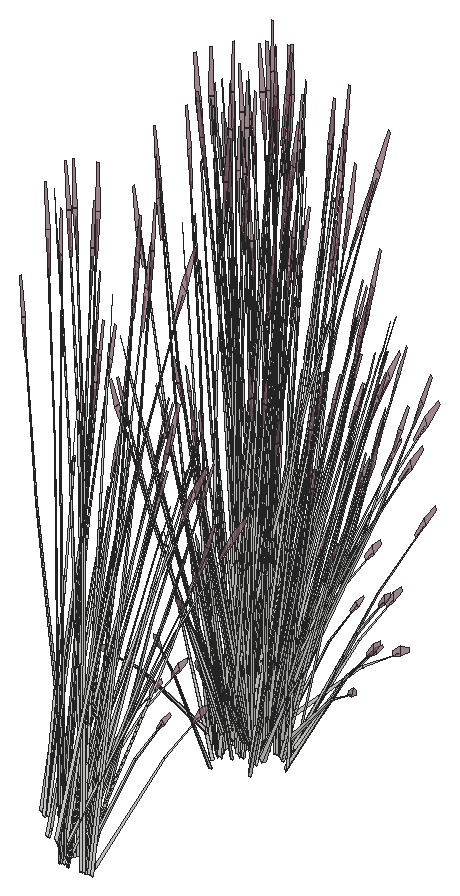
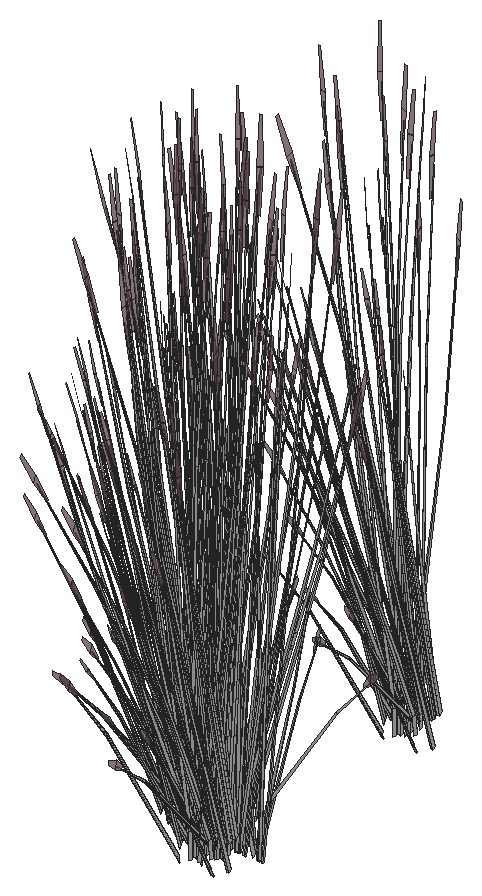
# SketchUp Ruby script. Lengths in inches.
U = 1.inch
M = Sketchup.active_model
def pt(a) = Geom::Point3d.new(a.map { |v| v * U })
def face(e, loops, mat)
  f = e.add_face(loops[0].map { |a| pt(a) })
  loops[1..].each { |l| e.add_face(l.map { |a| pt(a) }).erase! }
  f.material = f.back_material = mat if mat
  f
end
# faces: each face lists its corners as indices into pts; further lists are holes
def faces(e, pts, list, mat = nil) = list.each { |f| face(e, (f[0].is_a?(Array) ? f : [f]).map { |l| l.map { |i| pts[i] } }, mat) }
# xy, xz, yz: faces in a plane at the given z, y or x. An outline is a flat list of corners, or four numbers for a rectangle; further outlines are holes
def ring(l) = l.size == 4 ? [[l[0], l[1]], [l[2], l[1]], [l[2], l[3]], [l[0], l[3]]] : l.each_slice(2).to_a
def flat(e, list, mat, &to3) = list.each { |f| face(e, (f[0].is_a?(Array) ? f : [f]).map { |l| ring(l).map { |u, v| to3.(u, v) } }, mat) }
def xy(e, z, list, mat = nil) = flat(e, list, mat) { |x, y| [x, y, z] }
def xz(e, y, list, mat = nil) = flat(e, list, mat) { |x, z| [x, y, z] }
def yz(e, x, list, mat = nil) = flat(e, list, mat) { |y, z| [x, y, z] }
def lines(e, pts, list) = list.each { |a, b| e.add_line(pt(pts[a]), pt(pts[b])) }
# prism: a flat outline (further loops are holes) pulled along v
def prism(e, loops, v, mat = nil)
  f = face(e, loops, mat); d = Geom::Vector3d.new(v.map { |x| x * U })
  f.pushpull(f.normal.samedirection?(d) ? d.length : -d.length)
end
def box(e, o, s, mat = nil) = prism(e, [[o, [o[0] + s[0], o[1], o[2]], [o[0] + s[0], o[1] + s[1], o[2]], [o[0], o[1] + s[1], o[2]]]], [0, 0, s[2]], mat)
def at(x, y, z, deg = 0) = Geom::Transformation.translation(pt([x, y, z])) * Geom::Transformation.rotation(ORIGIN, Z_AXIS, deg.degrees)
def axes(o, x, y, z) = Geom::Transformation.new([*x, 0, *y, 0, *z, 0, *pt(o).to_a, 1])
def part(name) = M.definitions.add(name)
# library, detail: a bought-in or finely detailed component or shape, given as its bounding box
def library(name, o, s) = part(name).tap { |d| box(d.entities, o, s) }
def detail(e, o, s) = box(e.add_group.entities, o, s)
def put(e, d, t, mat = nil) = e.add_instance(d, t).tap { |i| i.material = mat if mat }
def group(e, t, mat = nil) = e.add_group.tap { |g| g.transformation = t; g.material = mat if mat }.entities
root = M.entities
M.materials.add("LightPink_Translucent").color = [144, 107, 117]
M.materials["LightPink_Translucent"].alpha = 0.75
c1 = part("blade")
p = [[2.15,0.21,22],[0,0.17,0],[0.09,0.45,0],[2.18,0.31,22],[2.29,0.31,22],[0.38,0.45,0],
  [2.48,0.24,33],[2.49,0.24,33],[2.48,0.22,33]]
faces(c1.entities,p,[[0,1,2,3],[4,5,2,3],[6,3,4,7],[8,0,3,6]])
c2 = part("seeds")
p = [[0.3,-0.1,1.38],[-0.01,-0.03,1.59],[-0.01,-0.03,0.03],[0.14,-0.07,-0.07],[0.29,-0.03,3],[0.15,0.01,3.11]]
faces(c2.entities,p,[[0,1,2,3],[1,0,4,5]],"LightPink_Translucent")
c3 = part("blade with seeds")
put(c3.entities,c1,at(0,0,0))
put(c3.entities,c2,axes([2.4,0.25,30.99],[1.5799,-0.05474,1.17369],[-0.12525,1.92788,0.29478],[-0.07173,-0.02425,1.56792]))
put(root,c3,axes([507.94,523.07,1.67],[0.7111,-0.30552,0.49651],[0.42504,0.54784,0],[-0.16196,0.06958,1.57504]))
put(root,c3,axes([506.93,522.59,1.48],[0.33034,0.70197,-0.06012],[-0.94388,0.24598,0],[0.01154,0.02451,1.72173]))
put(root,c3,axes([507.3,523.35,1.22],[-0.70886,-0.15119,-0.30978],[0.17848,-0.53243,0.30978],[-0.1429,0.0614,1.38974]))
put(root,c3,axes([510.04,521.32,1.57],[0.95008,0,0],[0,0.68292,-0.51607],[0,0.15554,1.63711]))
put(root,c3,axes([509.66,521.67,1.39],[-0.94962,-0.00489,-0.04976],[0,-0.68292,0.49943],[-0.02984,0.15546,1.58352]))
put(root,c3,axes([507.6,521.07,1.86],[0.85568,0.29155,-0.29095],[-0.41201,0.61537,-0.50002],[0.02689,0.15109,1.59708]))
put(root,c3,axes([509.26,522.83,3.72],[0.43232,0.38257,-0.35414],[-0.49364,0.36215,0.4572],[0.25081,0.0551,0.87481]))
put(root,c3,axes([509.46,521.77,1.22],[-0.53038,0.38124,-0.30978],[-0.53038,-0.38124,0.30978],[0,0.1228,1.38974]))
put(root,c3,axes([507.18,521.8,1.86],[0.08854,0.69723,-0.29095],[-0.92215,0.04216,-0.50002],[-0.16238,0.09287,1.59708]))
put(root,c3,axes([509.03,522.98,3.92],[-0.03826,0.46465,0.0643],[-0.57772,-0.01274,0.50621],[0.2213,0.04862,0.77189]))
put(root,c3,axes([507.51,521.53,1.4],[-0.36864,0.55059,-0.44739],[-0.76598,-0.26498,0.21531],[0,0.12692,1.43643]))
put(root,c3,axes([509.09,522.83,3.93],[-0.56024,0.40262,0.48003],[-0.48318,-0.42758,0.3958],[0.26285,0.07427,0.9933]))
put(root,c3,axes([507.31,523.29,4.24],[-0.11735,-0.49217,0.35414],[0.67083,-0.12996,-0.4572],[0.18018,0.14104,0.87481]))
put(root,c3,axes([507.53,523.11,1.52],[0.95122,0.19861,0.30756],[-0.23797,0.7099,-0.36492],[-0.15744,0.08885,1.64885]))
put(root,c3,axes([509.83,521.78,1.21],[0,0.61104,-0.49651],[-0.85008,0,0],[0,0.13917,1.57504]))
put(root,c3,axes([507.7,521.85,3.07],[-0.28223,-0.10528,1.71376],[0.58406,-0.44165,0.13857],[0.36402,0.19924,0.73262]))
put(root,c3,axes([507.76,520.46,3.67],[-0.65655,-0.31748,1.38283],[0.69326,-0.49431,0.59665],[0.21183,0.29789,1.33663]))
put(root,c3,axes([508.75,523.05,1.96],[-0.4278,-0.1757,1.1486],[0.5524,-0.17852,0.84392],[0.14899,0.15122,0.25299]))
put(root,c3,axes([507.24,523.55,4.23],[0.45276,-0.52302,-0.1216],[0.65568,0.30132,-0.67495],[0.22792,0.14777,1.02557]))
put(root,c3,axes([504.26,522.84,4.24],[0.5141,-0.32171,0.35414],[0.48666,0.36734,-0.4572],[-0.07405,0.18664,0.87481]))
put(root,c3,axes([508.11,523.49,1.57],[0.47504,0.61229,0],[-0.79476,0.34146,-0.51607],[-0.18101,0.07777,1.63711]))
put(root,c3,axes([506.65,523.98,3.9],[0.00225,-0.07398,1.77383],[0.65113,-0.32638,-0.16761],[0.22617,0.1165,0.31391]))
put(root,c3,axes([508.87,523.7,0.6875],[0.05536,-0.08822,1.76342],[0.69692,-0.25981,-0.26939],[0.21129,0.13447,0.30037]))
put(root,c3,axes([507.71,521.07,2.03],[-0.02076,-0.57531,1.41272],[0.93937,0.14913,0.59816],[-0.22217,0.31481,1.3335]))
put(root,c3,axes([507.95,521.7,1.29],[0.2786,0.55945,-0.69212],[-0.80253,0.20149,-0.18165],[0.03079,0.18945,1.52773]))
put(root,c3,axes([507.78,523.29,3.875],[0.74975,-0.14525,-0.51099],[0.13115,0.55007,-0.3958],[0.20138,0.15763,0.97773]))
put(root,c3,axes([505.7,523.37,4.24],[0.22906,-0.4699,0.35414],[0.66828,0.13705,-0.4572],[0.06128,0.18919,0.87481]))
put(root,c3,axes([508.82,523.85,1.86],[-0.48723,-0.01916,1.0506],[0.32177,-0.40701,0.58006],[0.19248,0.1446,0.8241]))
put(root,c3,axes([507.41,523.74,3.92],[-0.34533,0.38816,0.0643],[-0.49176,-0.22599,0.50621],[0.15898,0.12445,0.77189]))
put(root,c3,axes([506.6,525.05,4.84],[0.52505,-0.35054,-0.06488],[0.48109,0.38392,-0.29416],[0.03387,0.10878,0.97024]))
put(root,c3,axes([507.56,523.63,3.93],[-0.75571,0.14023,0.48003],[-0.13115,-0.55007,0.3958],[0.17773,0.16212,0.9933]))
put(root,c3,axes([507.22,522.86,1.78],[0.01341,-0.20255,1.43002],[0.64074,-0.22625,-0.30754],[0.1978,0.24243,0.61141]))
put(root,c3,axes([505.49,523.8,3.92],[-0.55987,0.20767,0.0643],[-0.27403,-0.37869,0.50621],[0.05407,0.16693,0.77189]))
put(root,c3,axes([503.93,522.93,4.59],[0.83505,0.03027,-0.13498],[-0.02282,0.57322,-0.74919],[-0.05801,0.22077,1.13838]))
put(root,c3,axes([505.48,523.57,4.23],[0.74352,-0.28449,-0.1216],[0.36538,0.50492,-0.67495],[0.0981,0.21277,1.02557]))
put(root,c3,axes([505.69,523.76,4.26],[-0.74868,-0.15974,0.53283],[0.25601,-0.52518,0.43934],[0.04499,0.20653,1.10256]))
put(root,c3,axes([505.61,523.68,0.6875],[0.12297,-0.03325,1.76342],[0.73967,0.18301,-0.26939],[0.02163,0.20626,0.30037]))
put(root,c3,axes([504.5,523.15,4.2],[0.54391,0.41056,-0.5672],[-0.57458,0.35956,-0.43934],[-0.08276,0.2086,1.08528]))
put(root,c3,axes([503.91,523.76,2.02],[0.69024,-0.1082,0.06507],[0.15868,0.43593,-0.86304],[-0.04376,0.22067,0.7736]))
put(root,c3,axes([506.12,523.54,3.875],[0.7469,0.15318,-0.51099],[-0.25601,0.52518,-0.3958],[0.06849,0.21144,0.97773]))
put(root,c3,axes([506.54,522.46,3.07],[-0.17368,-0.19618,1.71376],[0.80256,-0.16516,0.13857],[0.18139,0.30799,0.73262]))
put(root,c3,axes([505.78,523.87,3.72],[-0.22906,0.4699,-0.35414],[-0.66828,-0.13705,0.4572],[0.06128,0.18919,0.87481]))
put(root,c3,axes([505.12,522.56,3.07],[-0.0186,-0.23452,1.71376],[0.80601,0.15558,0.13857],[-0.04985,0.33422,0.73262]))
put(root,c3,axes([505.84,523.44,4.17],[0.36264,0.49684,-0.71045],[-0.74649,0.27689,0.08574],[0.0848,0.24006,1.00501]))
put(root,c3,axes([505.3,524.7,3.91],[0.09631,0.0984,1.74944],[0.77725,0.03866,-0.27667],[0.07816,0.217,0.14031]))
put(root,c3,axes([506.09,541.57,3.91],[-0.11621,-0.08567,1.74944],[-0.77555,0.05431,-0.27667],[-0.12378,-0.20491,0.14031]))
put(root,c3,axes([507.89,542.59,1.78],[-0.21597,0.12368,1.43002],[-0.64681,-0.21647,-0.30754],[0.1199,-0.26922,0.61141]))
put(root,c3,axes([506.9,543.02,4.17],[-0.36264,-0.49684,-0.71045],[0.74649,-0.27689,0.08574],[-0.0848,-0.24006,1.00501]))
put(root,c3,axes([506.28,541.91,0.6875],[-0.12744,0.02202,1.76342],[-0.70477,-0.24781,-0.26939],[0.01183,-0.2067,0.30037]))
put(root,c3,axes([508.41,543.5,4.17],[0.01977,-0.56521,-0.71045],[0.83252,0.03796,0.08574],[0.08786,-0.23945,1.00501]))
put(root,c3,axes([509.57,542.62,3.91],[-0.00733,-0.12161,1.74944],[-0.61946,-0.35147,-0.27667],[0.09577,-0.21306,0.14031]))
put(root,c3,axes([506.97,542.59,3.72],[0.22906,-0.4699,-0.35414],[0.66828,0.13705,0.4572],[-0.06128,-0.18919,0.87481]))
put(root,c3,axes([507.47,543.22,3.07],[-0.14147,0.21002,1.71376],[-0.59349,-0.43464,0.13857],[0.26773,-0.27089,0.73262]))
put(root,c3,axes([509.41,542.18,3.9],[-0.07716,0.04667,1.77383],[-0.75601,-0.15746,-0.16761],[-0.02737,-0.20368,0.31391]))
put(root,c3,axes([506.63,542.92,3.875],[-0.7469,-0.15318,-0.51099],[0.25601,-0.52518,-0.3958],[-0.06849,-0.21144,0.97773]))
put(root,c3,axes([507.09,541.6,1.96],[0.09747,0.35631,1.1486],[-0.54071,-0.19735,0.84392],[0.05818,-0.18244,0.25299]))
put(root,c3,axes([508.24,543.31,3.875],[-0.54391,-0.41056,-0.51099],[0.57458,-0.35956,-0.3958],[0.08276,-0.2086,0.97773]))
put(root,c3,axes([507.05,542.7,3.93],[0.74868,0.15974,0.48003],[-0.25601,0.52518,0.3958],[-0.04499,-0.20653,0.9933]))
put(root,c3,axes([507.27,542.89,4.23],[-0.74352,0.28449,-0.1216],[-0.36538,-0.50492,-0.67495],[-0.0981,-0.21277,1.02557]))
put(root,c3,axes([508.8125,543.53,4.23],[-0.83505,-0.03027,-0.1216],[0.02282,-0.57322,-0.67495],[0.05801,-0.22077,1.02557]))
put(root,c3,axes([508.75,543.16,3.72],[0.5141,-0.32171,-0.35414],[0.48666,0.36734,0.4572],[0.07405,-0.18664,0.87481]))
put(root,c3,axes([507.25,542.66,3.92],[0.55987,-0.20767,0.0643],[0.27403,0.37869,0.50621],[-0.05407,-0.16693,0.77189]))
put(root,c3,axes([505.22,544.88,1.29],[-0.31203,-0.62659,-0.69835],[0.89884,-0.22566,-0.18329],[-0.03449,-0.21218,1.54149]))
put(root,c3,axes([509.4,542.97,0.6875],[-0.11372,-0.04814,1.76342],[-0.29211,-0.53779,-0.26939],[0.19706,-0.14594,0.30037]))
put(root,c3,axes([507.04,543.09,4.24],[-0.22906,0.4699,0.35414],[-0.66828,-0.13705,-0.4572],[-0.06128,-0.18919,0.87481]))
put(root,c3,axes([508.75,543.29,3.93],[0.54105,0.41691,0.48003],[-0.57458,0.35956,0.3958],[0.0998,-0.1956,0.9933]))
put(root,c3,axes([508.95,543.33,3.92],[0.62439,0.02847,0.0643],[-0.01712,0.42991,0.50621],[0.06534,-0.16468,0.77189]))
put(root,c3,axes([508.49,543.62,4.24],[-0.5141,0.32171,0.35414],[-0.48666,-0.36734,-0.4572],[0.07405,-0.18664,0.87481]))
put(root,c3,axes([509.39,544.49,4.17],[0.39688,-0.48213,-0.71045],[0.69548,0.34264,0.08574],[0.23697,-0.17468,1.00501]))
put(root,c3,axes([505.1,543.08,1.57],[-0.47504,-0.61229,0],[0.79476,-0.34146,-0.51607],[0.18101,-0.07777,1.63711]))
put(root,c3,axes([509.37,544.26,3.875],[-0.19519,-0.55794,-0.51099],[0.73919,-0.0976,-0.3958],[0.21183,-0.14986,0.97773]))
put(root,c3,axes([506.14,542.34,1.32],[-0.52505,0.35054,-0.03893],[-0.48109,-0.38392,-0.17649],[-0.03387,-0.10878,0.58215]))
put(root,c3,axes([509.72,544.66,4.23],[-0.70283,-0.33692,-0.1216],[0.40491,-0.48793,-0.67495],[0.19857,-0.16961,1.02557]))
put(root,c3,axes([503.38,544.8,1.21],[0,-0.61104,-0.49651],[0.85008,0,0],[0,-0.13917,1.57504]))
put(root,c3,axes([505.75,542.99,1.21],[0.7111,-0.30552,-0.49651],[0.42504,0.54784,0],[0.16196,-0.06958,1.57504]))
put(root,c3,axes([509.97,544.04,1.78],[-0.27143,-0.0181,1.43002],[-0.27808,-0.48551,-0.30754],[0.33346,-0.13735,0.61141]))
put(root,c3,axes([511.45,544.51,3.9],[-0.09924,-0.00464,1.77383],[-0.4121,-0.49725,-0.16761],[0.1655,-0.1635,0.31391]))
put(root,c3,axes([506.59,544.24,1.25],[0.51177,-0.45928,-0.62353],[0.63575,0.41646,-0.16365],[0.20507,-0.11457,1.37633]))
put(root,c3,axes([510.28,543.15,1.96],[-0.25308,0.31105,1.1486],[-0.21753,-0.4179,0.84392],[0.20902,-0.10472,0.25299]))
put(root,c3,axes([509.92,544.32,3.72],[0.66138,-0.08733,-0.35414],[0.17464,0.49921,0.4572],[0.18953,-0.13408,0.87481]))
put(root,c3,axes([505.7,545.04,1.4],[0.36864,-0.55059,-0.44739],[0.76598,0.26498,0.21531],[0,-0.12692,1.43643]))
put(root,c3,axes([506.04,544.77,1.86],[-0.08854,-0.69723,-0.29095],[0.92215,-0.04216,-0.50002],[0.16238,-0.09287,1.59708]))
put(root,c3,axes([503.75,544.81,1.22],[0.53038,-0.38124,-0.30978],[0.53038,0.38124,0.30978],[0,-0.1228,1.38974]))
put(root,c3,axes([509.38,544.61,4.24],[-0.66138,0.08733,0.35414],[-0.17464,-0.49921,-0.4572],[0.18953,-0.13408,0.87481]))
put(root,c3,axes([505.61,545.5,1.86],[-0.85568,-0.29155,-0.29095],[0.41201,-0.61537,-0.50002],[-0.02689,-0.15109,1.59708]))
put(root,c3,axes([505.91,543.23,1.22],[0.70886,0.15119,-0.30978],[-0.17848,0.53243,0.30978],[0.1429,-0.0614,1.38974]))
put(root,c3,axes([509.98,544.53,3.92],[0.52161,0.25698,0.0643],[-0.30368,0.36595,0.50621],[0.16723,-0.11831,0.77189]))
put(root,c3,axes([509.83,544.43,3.93],[0.18844,0.56237,0.48003],[-0.73919,0.0976,0.3958],[0.21785,-0.13226,0.9933]))
put(root,c3,axes([511.83,545.11,3.91],[0.10543,-0.09307,1.74944],[-0.13495,-0.57092,-0.27667],[0.26455,-0.10825,0.14031]))
put(root,c3,axes([506.16,545.32,1.625],[0.8561,0.29616,0.24065],[-0.41201,0.61537,0.50002],[0,-0.14185,1.60543]))
put(root,c3,axes([505.88,544.91,1.91],[-0.82508,0.03772,0.44739],[-0.07462,-0.62614,-0.21531],[0.14771,-0.06346,1.43643]))
put(root,c3,axes([503.75,545.36,1.67],[0,0.61104,0.49651],[-0.85008,0,0],[0,-0.13917,1.57504]))
put(root,c3,axes([509.75,545.97,4.23],[-0.38229,-0.5533,-0.1216],[0.6785,-0.2719,-0.67495],[0.28593,-0.073,1.02557]))
put(root,c3,axes([509.72,545.5,3.875],[0.20584,-0.55581,-0.51099],[0.70573,0.19051,-0.3958],[0.28414,-0.05097,0.97773]))
put(root,c3,axes([508.6,543.24,1.57],[0.47504,-0.61229,0],[0.79476,0.34146,-0.51607],[0.18101,0.07777,1.63711]))
put(root,c3,axes([505.85,545.13,1.55],[0.33034,0.68327,0.45755],[-0.94388,0.2376,0.17955],[0.01154,-0.12555,1.58856]))
put(root,c3,axes([510.47,545.66,1.17],[-0.48937,0.07333,1.41583],[-0.07789,-0.58369,0.08104],[0.34275,-0.08835,0.80566]))
put(root,c3,axes([511.36,545.14,1.45],[-0.47106,-0.39072,-0.06488],[0.51591,-0.35801,-0.29416],[0.14618,-0.02521,0.97024]))
put(root,c3,axes([505.68,545.67,1.91],[-0.36864,0.55059,0.44739],[-0.76598,-0.26498,-0.21531],[0,-0.12692,1.43643]))
put(root,c3,axes([507.04,545.1875,1.4],[0,-0.70701,0],[0.95008,0,0],[0,0,1.79456]))
put(root,c3,axes([508.19,543.56,1.67],[-0.7111,-0.30552,0.49651],[0.42504,-0.54784,0],[0.16196,0.06958,1.57504]))
put(root,c3,axes([509.58,545.7,4.17],[0.66765,-0.26986,-0.71045],[0.37208,0.55551,0.08574],[0.32259,-0.0631,1.00501]))
put(root,c3,axes([506.59,544.74,1.55],[-0.62999,0.55453,0.45755],[-0.74845,-0.4895,0.17955],[0.15188,-0.05534,1.58856]))
put(root,c3,axes([507.28,545.74,1.49],[-0.70674,-0.52593,-0.06131],[0.70717,-0.52625,0],[-0.02468,-0.01837,1.75571]))
put(root,c3,axes([505.49,543.83,1.67],[-0.21949,0.60727,0.17642],[-0.8032,-0.17185,0.35086],[0.13875,-0.00296,1.60407]))
put(root,c3,axes([509.48,545.81,4.24],[-0.63144,-0.17046,0.35414],[0.18417,-0.49731,-0.4572],[0.25423,-0.0456,0.87481]))
put(root,c3,axes([505.16,544.32,0.79],[-0.74787,0.24464,1.28929],[-0.23804,-0.70192,0.50096],[0.45924,0.01168,1.46642]))
put(root,c3,axes([507.17,544.51,1.81],[0.14658,-0.54532,0.1448],[0.71613,0.09466,-0.41347],[0.13033,0.05599,1.26744]))
put(root,c3,axes([505.93,545.8,1.55],[0.96033,0.12874,0.45755],[-0.19544,0.7271,0.17955],[-0.14034,-0.07021,1.58856]))
put(root,c3,axes([511,545.27,0.6875],[-0.03971,-0.09277,1.76342],[0.27541,-0.54264,-0.26939],[0.27782,-0.00781,0.30037]))
put(root,c3,axes([506.87,544.65,1.91],[-0.45644,-0.51287,0.44739],[0.69137,-0.36116,-0.21531],[0.14771,0.06346,1.43643]))
put(root,c3,axes([505.42,546.96,1.67],[0.81646,-0.16218,0.17642],[0.20161,0.60355,0.35086],[-0.07282,-0.08794,1.60407]))
put(root,c3,axes([507.1,544.68,1.86],[0.76714,-0.40567,-0.29095],[0.51013,0.57321,-0.50002],[0.18927,0.05821,1.59708]))
put(root,c3,axes([510.15,545.75,3.72],[0.63144,0.17046,-0.35414],[-0.18417,0.49731,0.4572],[0.25423,-0.0456,0.87481]))
put(root,c3,axes([509.03,543.6,1.21],[0.7111,0.30552,-0.49651],[-0.42504,0.54784,0],[0.16196,0.06958,1.57504]))
put(root,c3,axes([507.68,545.35,1.4],[0.85008,0,0],[0,0.63259,0],[0,0,1.78407]))
put(root,c3,axes([507.92,543.86,1.67],[-0.81646,0.16218,0.17642],[-0.20161,-0.60355,0.35086],[0.07282,0.08794,1.60407]))
put(root,c3,axes([508.43,545.14,3.07],[-0.31515,0.01384,1.71376],[0.20907,-0.5998,0.13857],[0.44912,0.0371,0.73262]))
put(root,c3,axes([508.83,543.83,1.22],[0.17848,0.53243,-0.30978],[-0.70886,0.15119,0.30978],[0.1429,0.0614,1.38974]))
put(root,c3,axes([510.06,545.96,3.92],[0.27906,0.41663,0.0643],[-0.50888,0.20393,0.50621],[0.22432,-0.04024,0.77189]))
put(root,c3,axes([507.41,545.03,1.57],[-0.96033,-0.12874,0.49198],[0.19544,-0.7271,0.19306],[0.14034,0.07021,1.70813]))
put(root,c3,axes([510,545.8125,3.93],[-0.21466,0.55714,0.48003],[-0.70573,-0.19051,0.3958],[0.27753,-0.03348,0.9933]))
put(root,c3,axes([506.64,546.82,1.4],[-0.24791,-0.5268,0],[0.70791,-0.18448,0],[0,0,1.54371]))
put(root,c3,axes([507.57,546.75,1.38],[0.79769,-0.20732,-0.19198],[0.2803,0.59721,0.00008],[0.08805,-0.02292,1.73897]))
put(root,c3,axes([507.85,547,1.67],[0.21949,-0.60727,0.17642],[0.8032,0.17185,0.35086],[-0.13875,0.00296,1.60407]))
put(root,c3,axes([507.66,545.62,1.41],[0.53038,0.39469,0],[-0.53038,0.39469,0],[0,0,1.69266]))
put(root,c3,axes([509.1,545.45,1.67],[-0.59697,-0.44509,0.17642],[0.60159,-0.4317,0.35086],[-0.06593,0.0909,1.60407]))
put(root,c3,axes([508,544.77,1.25],[0.79037,0.10018,-0.62353],[-0.16679,0.61794,-0.16365],[0.23587,0.07488,1.37633]))
put(root,c3,axes([511.49,545.85,1.96],[-0.46945,0.10088,1.1486],[0.22097,-0.4169,0.84392],[0.24904,0.02853,0.25299]))
put(root,c3,axes([506.47,547.06,1.39],[-0.76598,-0.27433,0],[0.36864,-0.57001,0],[0,0,1.62707]))
put(root,c3,axes([507.66,545.16,1.91],[0.36864,-0.55059,0.44739],[0.76598,0.26498,-0.21531],[0,0.12692,1.43643]))
put(root,c3,axes([511.27,547.62,3.9],[-0.0687,-0.05349,1.77383],[0.15029,-0.57341,-0.16761],[0.27062,-0.03664,0.31391]))
put(root,c3,axes([507.52,545.47,1.48],[0,0.70667,-0.05637],[-0.95008,0,0],[0,0.02221,1.79368]))
put(root,c3,axes([507.59,544.97,1.4],[0.45644,0.51287,-0.44739],[-0.69137,0.36116,0.21531],[0.14771,0.06346,1.43643]))
put(root,c3,axes([510.67,547.14,3.12],[-0.14542,-0.51365,-0.03492],[0.68734,-0.11809,-0.15832],[0.14353,0.03256,0.52218]))
put(root,c3,axes([508.89,547.125,4.23],[0.04068,-0.62141,-0.1216],[0.77029,0.01698,-0.67495],[0.29667,0.04317,1.02557]))
put(root,c3,axes([509.59,545.46,1.67],[0,-0.61104,0.49651],[0.85008,0,0],[0,0.13917,1.57504]))
put(root,c3,axes([507.46,545.92,1.91],[0.82508,-0.03772,0.44739],[0.07462,0.62614,-0.21531],[-0.14771,0.06346,1.43643]))
put(root,c3,axes([507.98,545.28,1.81],[0.70791,-0.1782,0.1448],[0.24791,0.50885,-0.41347],[0,0.11199,1.26744]))
put(root,c3,axes([508.77,546.88,4.24],[-0.43232,-0.38257,0.35414],[0.49364,-0.36215,-0.4572],[0.25081,0.0551,0.87481]))
put(root,c3,axes([510.61,546.52,1.78],[-0.18299,-0.15028,1.43002],[0.23809,-0.49714,-0.30754],[0.37023,0.06735,0.61141]))
put(root,c3,axes([507.34,547.07,1.4],[0.76598,0.27433,0],[-0.36864,0.57001,0],[0,0,1.74954]))
put(root,c3,axes([509.5625,546.75,3.91],[0.16299,-0.01033,1.74944],[0.44707,-0.47471,-0.27667],[0.28992,0.06266,0.14031]))
put(root,c3,axes([507.64,547.68,1.39],[-0.46912,-0.61443,-0.05142],[0.79476,-0.34146,0.51607],[-0.19584,0.0585,1.6363]))
put(root,c3,axes([507.48,546.19,1.81],[0.56134,0.36712,0.1448],[-0.46823,0.41419,-0.41347],[-0.13033,0.05599,1.26744]))
put(root,c3,axes([508.93,546.82,4.17],[0.75952,0.01471,-0.71045],[-0.05101,0.61953,0.08574],[0.32177,0.06538,1.00501]))
put(root,c3,axes([508.07,547.32,1.67],[0.7111,-0.30552,0.49651],[0.42504,0.54784,0],[-0.16196,0.06958,1.57504]))
put(root,c3,axes([507.0625,546.84,1.48],[0.33034,0.70197,-0.06012],[-0.94388,0.24598,0],[0.01154,0.02451,1.72173]))
put(root,c3,axes([507.43,547.6,1.22],[-0.70886,-0.15119,-0.30978],[0.17848,-0.53243,0.30978],[-0.1429,0.0614,1.38974]))
put(root,c3,axes([510.17,545.57,1.57],[0.95008,0,0],[0,0.68292,-0.51607],[0,0.15554,1.63711]))
put(root,c3,axes([509.79,545.92,1.39],[-0.94962,-0.00489,-0.04976],[0,-0.68292,0.49943],[-0.02984,0.15546,1.58352]))
put(root,c3,axes([507.74,545.32,1.86],[0.85568,0.29155,-0.29095],[-0.41201,0.61537,-0.50002],[0.02689,0.15109,1.59708]))
put(root,c3,axes([509.39,547.08,3.72],[0.43232,0.38257,-0.35414],[-0.49364,0.36215,0.4572],[0.25081,0.0551,0.87481]))
put(root,c3,axes([509.59,546.02,1.22],[-0.53038,0.38124,-0.30978],[-0.53038,-0.38124,0.30978],[0,0.1228,1.38974]))
put(root,c3,axes([507.31,546.05,1.86],[0.08854,0.69723,-0.29095],[-0.92215,0.04216,-0.50002],[-0.16238,0.09287,1.59708]))
put(root,c3,axes([509.16,547.23,3.92],[-0.03826,0.46465,0.0643],[-0.57772,-0.01274,0.50621],[0.2213,0.04862,0.77189]))
put(root,c3,axes([507.64,545.78,1.4],[-0.36864,0.55059,-0.44739],[-0.76598,-0.26498,0.21531],[0,0.12692,1.43643]))
put(root,c3,axes([509.22,547.08,3.93],[-0.56024,0.40262,0.48003],[-0.48318,-0.42758,0.3958],[0.26285,0.07427,0.9933]))
put(root,c3,axes([507.4375,547.54,4.24],[-0.11735,-0.49217,0.35414],[0.67083,-0.12996,-0.4572],[0.18018,0.14104,0.87481]))
put(root,c3,axes([507.66,547.36,1.52],[0.95122,0.19861,0.30756],[-0.23797,0.7099,-0.36492],[-0.15744,0.08885,1.64885]))
put(root,c3,axes([507.6,547.84,1.21],[-0.7111,0.30552,-0.49651],[-0.42504,-0.54784,0],[-0.16196,0.06958,1.57504]))
put(root,c3,axes([509.96,546.03,1.21],[0,0.61104,-0.49651],[-0.85008,0,0],[0,0.13917,1.57504]))
put(root,c3,axes([507.83,546.1,3.07],[-0.28223,-0.10528,1.71376],[0.58406,-0.44165,0.13857],[0.36402,0.19924,0.73262]))
put(root,c3,axes([507.89,544.71,3.67],[-0.65655,-0.31748,1.38283],[0.69326,-0.49431,0.59665],[0.21183,0.29789,1.33663]))
put(root,c3,axes([508.88,547.3,1.96],[-0.4278,-0.1757,1.1486],[0.5524,-0.17852,0.84392],[0.14899,0.15122,0.25299]))
put(root,c3,axes([507.375,547.8,4.23],[0.45276,-0.52302,-0.1216],[0.65568,0.30132,-0.67495],[0.22792,0.14777,1.02557]))
put(root,c3,axes([504.39,547.09,4.24],[0.5141,-0.32171,0.35414],[0.48666,0.36734,-0.4572],[-0.07405,0.18664,0.87481]))
put(root,c3,axes([508.24,547.75,1.57],[0.47504,0.61229,0],[-0.79476,0.34146,-0.51607],[-0.18101,0.07777,1.63711]))
put(root,c3,axes([506.78,548.23,3.9],[0.00225,-0.07398,1.77383],[0.65113,-0.32638,-0.16761],[0.22617,0.1165,0.31391]))
put(root,c3,axes([509,547.95,0.6875],[0.05536,-0.08822,1.76342],[0.69692,-0.25981,-0.26939],[0.21129,0.13447,0.30037]))
put(root,c3,axes([507.84,545.32,2.03],[-0.02076,-0.57531,1.41272],[0.93937,0.14913,0.59816],[-0.22217,0.31481,1.3335]))
put(root,c3,axes([508.08,545.95,1.29],[0.2786,0.55945,-0.69212],[-0.80253,0.20149,-0.18165],[0.03079,0.18945,1.52773]))
put(root,c3,axes([507.91,547.54,3.875],[0.74975,-0.14525,-0.51099],[0.13115,0.55007,-0.3958],[0.20138,0.15763,0.97773]))
put(root,c3,axes([505.83,547.62,4.24],[0.22906,-0.4699,0.35414],[0.66828,0.13705,-0.4572],[0.06128,0.18919,0.87481]))
put(root,c3,axes([508.95,548.1,1.86],[-0.48723,-0.01916,1.0506],[0.32177,-0.40701,0.58006],[0.19248,0.1446,0.8241]))
put(root,c3,axes([507.54,547.99,3.92],[-0.34533,0.38816,0.0643],[-0.49176,-0.22599,0.50621],[0.15898,0.12445,0.77189]))
put(root,c3,axes([506.73,549.3,4.84],[0.52505,-0.35054,-0.06488],[0.48109,0.38392,-0.29416],[0.03387,0.10878,0.97024]))
put(root,c3,axes([507.6875,547.88,3.93],[-0.75571,0.14023,0.48003],[-0.13115,-0.55007,0.3958],[0.17773,0.16212,0.9933]))
put(root,c3,axes([507.35,547.11,1.78],[0.01341,-0.20255,1.43002],[0.64074,-0.22625,-0.30754],[0.1978,0.24243,0.61141]))
put(root,c3,axes([505.625,548.05,3.92],[-0.55987,0.20767,0.0643],[-0.27403,-0.37869,0.50621],[0.05407,0.16693,0.77189]))
put(root,c3,axes([504.0625,547.18,4.59],[0.83505,0.03027,-0.13498],[-0.02282,0.57322,-0.74919],[-0.05801,0.22077,1.13838]))
put(root,c3,axes([505.61,547.82,4.23],[0.74352,-0.28449,-0.1216],[0.36538,0.50492,-0.67495],[0.0981,0.21277,1.02557]))
put(root,c3,axes([505.82,548.01,4.26],[-0.74868,-0.15974,0.53283],[0.25601,-0.52518,0.43934],[0.04499,0.20653,1.10256]))
put(root,c3,axes([505.74,547.93,0.6875],[0.12297,-0.03325,1.76342],[0.73967,0.18301,-0.26939],[0.02163,0.20626,0.30037]))
put(root,c3,axes([504.63,547.4,4.2],[0.54391,0.41056,-0.5672],[-0.57458,0.35956,-0.43934],[-0.08276,0.2086,1.08528]))
put(root,c3,axes([504.04,548.01,2.02],[0.69024,-0.1082,0.06507],[0.15868,0.43593,-0.86304],[-0.04376,0.22067,0.7736]))
put(root,c3,axes([506.25,547.8,3.875],[0.7469,0.15318,-0.51099],[-0.25601,0.52518,-0.3958],[0.06849,0.21144,0.97773]))
put(root,c3,axes([506.67,546.71,3.07],[-0.17368,-0.19618,1.71376],[0.80256,-0.16516,0.13857],[0.18139,0.30799,0.73262]))
put(root,c3,axes([505.91,548.12,3.72],[-0.22906,0.4699,-0.35414],[-0.66828,-0.13705,0.4572],[0.06128,0.18919,0.87481]))
put(root,c3,axes([505.25,546.81,3.07],[-0.0186,-0.23452,1.71376],[0.80601,0.15558,0.13857],[-0.04985,0.33422,0.73262]))
put(root,c3,axes([505.97,547.7,4.17],[0.36264,0.49684,-0.71045],[-0.74649,0.27689,0.08574],[0.0848,0.24006,1.00501]))
put(root,c3,axes([505.43,548.95,3.91],[0.09631,0.0984,1.74944],[0.77725,0.03866,-0.27667],[0.07816,0.217,0.14031]))
